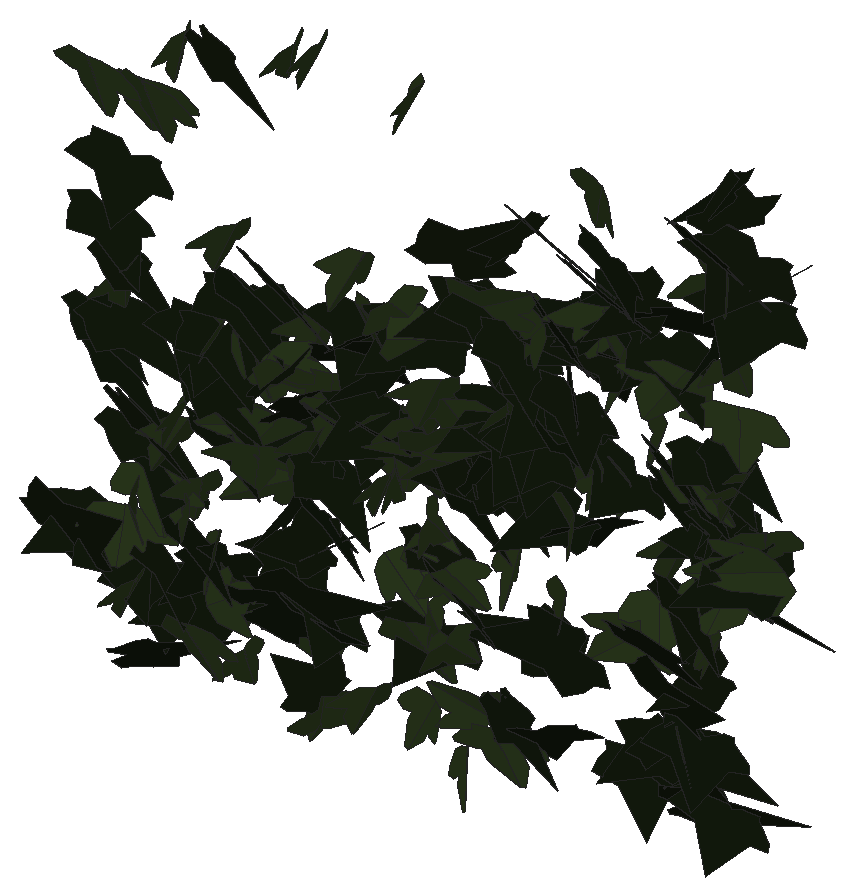
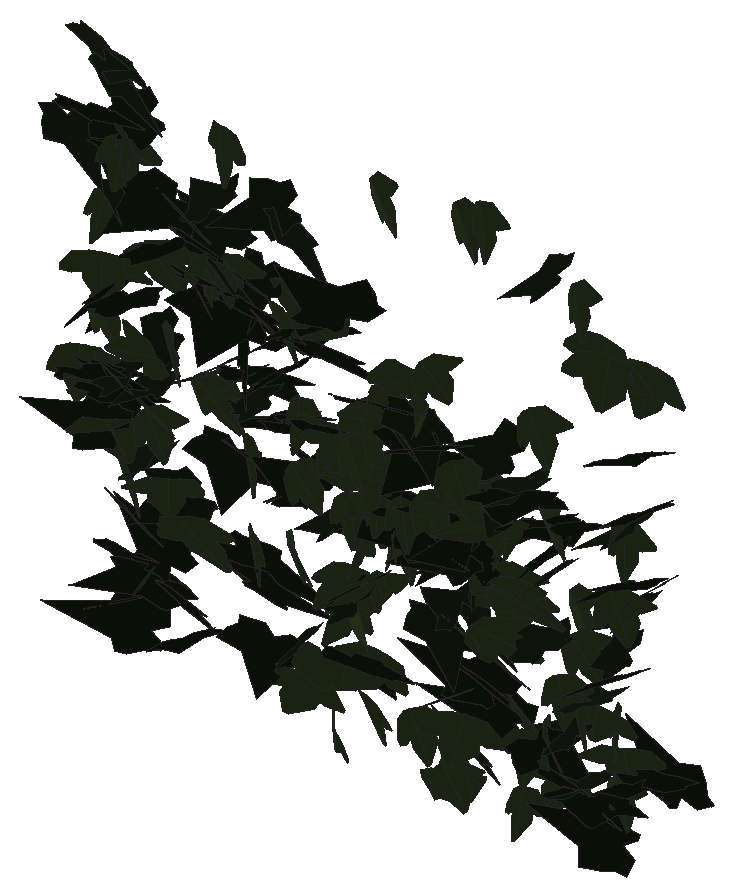
# SketchUp Ruby script. Lengths in millimetres.
U = 1.mm
M = Sketchup.active_model
def pt(a) = Geom::Point3d.new(a.map { |v| v * U })
def face(e, loops, mat)
  f = e.add_face(loops[0].map { |a| pt(a) })
  loops[1..].each { |l| e.add_face(l.map { |a| pt(a) }).erase! }
  f.material = f.back_material = mat if mat
  f
end
# faces: each face lists its corners as indices into pts; further lists are holes
def faces(e, pts, list, mat = nil) = list.each { |f| face(e, (f[0].is_a?(Array) ? f : [f]).map { |l| l.map { |i| pts[i] } }, mat) }
# xy, xz, yz: faces in a plane at the given z, y or x. An outline is a flat list of corners, or four numbers for a rectangle; further outlines are holes
def ring(l) = l.size == 4 ? [[l[0], l[1]], [l[2], l[1]], [l[2], l[3]], [l[0], l[3]]] : l.each_slice(2).to_a
def flat(e, list, mat, &to3) = list.each { |f| face(e, (f[0].is_a?(Array) ? f : [f]).map { |l| ring(l).map { |u, v| to3.(u, v) } }, mat) }
def xy(e, z, list, mat = nil) = flat(e, list, mat) { |x, y| [x, y, z] }
def xz(e, y, list, mat = nil) = flat(e, list, mat) { |x, z| [x, y, z] }
def yz(e, x, list, mat = nil) = flat(e, list, mat) { |y, z| [x, y, z] }
def lines(e, pts, list) = list.each { |a, b| e.add_line(pt(pts[a]), pt(pts[b])) }
# prism: a flat outline (further loops are holes) pulled along v
def prism(e, loops, v, mat = nil)
  f = face(e, loops, mat); d = Geom::Vector3d.new(v.map { |x| x * U })
  f.pushpull(f.normal.samedirection?(d) ? d.length : -d.length)
end
def box(e, o, s, mat = nil) = prism(e, [[o, [o[0] + s[0], o[1], o[2]], [o[0] + s[0], o[1] + s[1], o[2]], [o[0], o[1] + s[1], o[2]]]], [0, 0, s[2]], mat)
def at(x, y, z, deg = 0) = Geom::Transformation.translation(pt([x, y, z])) * Geom::Transformation.rotation(ORIGIN, Z_AXIS, deg.degrees)
def axes(o, x, y, z) = Geom::Transformation.new([*x, 0, *y, 0, *z, 0, *pt(o).to_a, 1])
def part(name) = M.definitions.add(name)
# library, detail: a bought-in or finely detailed component or shape, given as its bounding box
def library(name, o, s) = part(name).tap { |d| box(d.entities, o, s) }
def detail(e, o, s) = box(e.add_group.entities, o, s)
def put(e, d, t, mat = nil) = e.add_instance(d, t).tap { |i| i.material = mat if mat }
def group(e, t, mat = nil) = e.add_group.tap { |g| g.transformation = t; g.material = mat if mat }.entities
root = M.entities
M.materials.add("efeu1").color = [18, 25, 13]
M.materials.add("efeu2").color = [43, 57, 29]
c1 = part("ivyleaf_9")
p = [[39.1,54.8,31.7],[34.5,51.8,30.2],[-5.3,25.2,17.3],[-17.9,28.3,20.9],[-21.6,21.7,17],[-20.2,4.3,5.3],
  [-22.9,-0.3,2.5],[-17.1,-4,-0.6],[-2,-2.1,-1.2],[-0.7,-15.4,-10.1],[16.6,-22.3,-16.7],[21.1,-15.1,-12.5],
  [32.7,-10.7,-11],[46.1,-1.8,-6.6],[30.8,11.2,3.8]]
faces(c1.entities,p,[[0,1,2,3,4,5,6,7,8,9,10,11,12,13,14]],"efeu1")
c2 = part("ivyleaf_10")
p = [[0,12.8,-0.8],[-1.5,51.3,-10.9],[-4.9,51,-11.6],[-13.6,26.5,-7.3],[-13.2,15.9,-4.6],[-21.1,19.3,-7.2],
  [-29.5,16.3,-8.3],[-29.2,8.3,-6.2],[-19.7,-9.8,0.5],[-7.6,-13,4],[1,-12.2,5.8],[-0.4,51.1,-11.1],
  [-1.5,51.1,-10.9],[1,-12.4,5.9],[16.9,-12.4,3.5],[35.1,9.1,-5.1],[35,12.9,-6.1],[20.5,16.4,-4.9],
  [15.8,15,-3.8],[15.3,27.6,-7.1],[12.8,31.3,-7.8]]
faces(c2.entities,p,[[0,1,2,3,4,5,6,7,8,9,10],[11,12,0,13,14,15,16,17,18,19,20]],"efeu2")
put(root,c1,axes([4004.6,807.1,2723.3],[-1.72349,-0.38315,0.30559],[-0.51909,-0.13943,-0.98307],[0.77495,-0.94552,0.02113]))
put(root,c1,axes([3962.3,785.5,2704.8],[-0.47252,0.12478,1.19338],[1.21455,-1.01828,0.23923],[1.93387,0.67001,0.14134]))
put(root,c2,axes([4006,787.8,3291.4],[-2.04812,0.34445,-0.02824],[0.02425,-0.05275,-1.12898],[-0.65731,-1.07522,0.04634]))
put(root,c1,axes([3997.3,798.5,2991.7],[0.61956,-0.96621,-0.38496],[-0.14432,0.38025,-1.01852],[1.97419,0.33102,0.04636]))
put(root,c1,axes([4005.8,810.3,3106.3],[-0.00206,-1.09219,-0.16823],[0.07466,0.16809,-1.0915],[2.10184,-0.00704,0.03861]))
put(root,c2,axes([4038.1,819,2966.8],[-0.79231,-1.00282,0.18365],[0.00996,-0.20047,-1.08281],[1.94029,-0.40847,0.08055]))
put(root,c1,axes([4033.7,814.1,3176.8],[-0.91795,-0.98023,0.18834],[0.03143,-0.21698,-1.08702],[1.89944,-0.47013,0.109]))
put(root,c1,axes([4023.4,804,2703.1],[-0.20194,-1.01434,-0.32948],[0.12304,0.32438,-1.01946],[2.02605,-0.1208,0.02907]))
put(root,c2,axes([4035.6,801.1,2740.4],[1.71839,0.57529,-0.10566],[-0.18811,-0.04148,-1.07045],[-1.0972,0.90811,0.01804]))
put(root,c2,axes([4044.9,789.4,3049.4],[-0.37987,-1.03459,-0.33106],[0.16608,0.32024,-1.0534],[2.06071,-0.21653,0.02387]))
put(root,c1,axes([4024.5,788.4,2950.3],[0.88277,-0.96056,-0.20735],[-0.12452,0.19859,-1.06635],[1.8661,0.46765,0.02693]))
put(root,c1,axes([4025,799.5,2992.3],[0.4837,-0.85668,-0.61589],[0.28995,0.65666,-0.85053],[1.98701,0.11272,0.27404]))
put(root,c2,axes([4061,781,2676.1],[-0.15705,-1.01305,-0.15562],[-0.00419,0.1563,-1.0163],[1.95065,-0.08123,-0.01471]))
put(root,c2,axes([4070.3,776.8,2773.9],[-0.55798,0.64958,0.78832],[-0.92662,0.63213,-0.70194],[-1.70902,-0.55481,0.12321]))
put(root,c1,axes([4032.1,793.5,3068.4],[1.03234,-0.93965,-0.3083],[-0.04797,0.33838,-1.07568],[1.88153,0.52419,0.14173]))
put(root,c1,axes([4037.2,812.7,2858.8],[0.73316,-0.85605,-0.58965],[0.11836,0.64669,-0.89823],[1.97478,0.27906,0.27275]))
put(root,c2,axes([4073.6,795.2,3286.1],[-2.13847,-0.12835,0.03775],[-0.07317,0.00396,-1.1309],[0.24389,-1.12425,-0.00829]))
put(root,c1,axes([4039,797.4,2886.7],[1.24053,-0.8578,0.06357],[0.06334,-0.05455,-1.07733],[1.63581,0.65263,-0.0065]))
put(root,c1,axes([4077.4,822,2674.8],[-1.29878,-0.72357,-0.43124],[0.56055,0.315,-0.99461],[1.50194,-0.74326,-0.0017]))
put(root,c2,axes([4070.1,810.4,2795.4],[2.02443,-0.08077,0.312],[0.59043,-0.03493,-1.06671],[0.16619,1.10796,-0.01088]))
put(root,c1,axes([4081.3,827.1,2809.1],[-0.63423,-0.84696,0.56115],[0.15184,-0.61055,-0.87415],[1.92765,-0.23057,0.25348]))
put(root,c2,axes([4093,775.9,3296.1],[-2.00794,0.43932,-0.03649],[0.05659,-0.02351,-1.1428],[-0.83708,-1.0554,0.01027]))
put(root,c1,axes([4064.9,779.3,2592.2],[0.91622,0.90677,-0.46551],[0.34977,0.42916,1.02603],[1.90809,-0.51408,0.03545]))
put(root,c2,axes([4106.6,807.1,2876],[-0.38013,-1.01756,0.40443],[-0.0116,-0.41007,-1.03475],[2.08395,-0.18789,0.06801]))
put(root,c1,axes([4084.4,828,2688],[-0.26892,-0.97988,0.5077],[0.22139,-0.52221,-0.97552],[2.08866,-0.07081,0.16877]))
put(root,c2,axes([4117.7,798.6,2786.9],[0.89494,-0.78912,-0.53773],[-0.22852,0.54577,-0.90592],[1.80297,0.46087,0.15209]))
put(root,c2,axes([4124.4,787.2,3367.2],[0.08101,-1.14133,-0.10536],[0.22551,0.10925,-1.13559],[2.16973,0.03126,0.12196]))
put(root,c2,axes([4130.4,779.9,2920.2],[0.32381,-1.08677,0.02998],[0.00989,-0.02953,-1.10001],[2.0691,0.17022,0.00056]))
put(root,c2,axes([4130.6,811.7,2811.8],[-0.61298,-0.98323,-0.10761],[0.13937,0.08916,-1.03381],[1.8773,-0.32767,0.04161]))
put(root,c1,axes([4162.6,808.7,2679.1],[-2.03173,0.36853,0.09714],[-0.17909,0.02508,-1.12933],[-0.70289,-1.07165,0.00698]))
put(root,c1,axes([4109.2,813.4,2750.4],[0.60615,-1.00713,0.35708],[0.28831,-0.32628,-1.05539],[2.01314,0.34997,0.04363]))
put(root,c1,axes([4159.8,821.7,2725.4],[0.03041,0.38777,-0.98513],[0.05152,-0.98507,-0.38731],[-2.01427,-0.01934,-0.02478]))
put(root,c2,axes([4140,825.9,2736.1],[0.822,-0.72874,0.63942],[0.68113,-0.53071,-0.84659],[1.71481,0.56012,0.02976]))
put(root,c2,axes([4154.2,772,2652.5],[-1.80375,0.35185,-0.20836],[0.38987,-0.04667,-1.01059],[-0.67355,-0.96926,-0.02698]))
put(root,c1,axes([4163.6,791.5,3019.6],[-1.04671,-0.97554,0.10136],[-0.08043,-0.09253,-1.11985],[1.86491,-0.55153,0.00859]))
put(root,c2,axes([4173.8,786.2,3028.6],[0.66739,-1.03691,0.10548],[0.03954,-0.10431,-1.09452],[1.98324,0.35102,-0.01367]))
put(root,c1,axes([4146.9,827,2868.1],[0.20036,-0.89986,0.58289],[0.55983,-0.53898,-0.8852],[1.96223,0.24566,0.19303]))
put(root,c1,axes([4156.9,799.4,2958.2],[0.59458,-1.02655,-0.16373],[-0.05627,0.16212,-1.07287],[1.97763,0.31325,0.0187]))
put(root,c2,axes([4186.3,809.2,2706],[-1.62772,0.5965,0.21832],[-0.3537,0.11515,-1.04266],[-1.156,-0.87514,0.01161]))
put(root,c2,axes([4196.7,782.2,3158.7],[-0.47503,-1.11575,0.00757],[-0.03301,-0.00388,-1.14322],[2.12329,-0.24968,-0.01608]))
put(root,c1,axes([4173.9,773.7,2978.9],[0.73145,-0.84348,-0.68833],[-0.52372,0.63099,-0.92687],[2.00473,0.4726,0.00901]))
put(root,c1,axes([4167.4,779.6,3380.1],[1.24893,-0.93043,-0.21111],[-0.17753,0.19243,-1.13805],[1.8071,0.66194,0.0341]))
put(root,c2,axes([4223.1,809.6,2917.5],[1.11307,-0.02398,-0.89333],[-1.67782,0.15942,-0.58143],[0.27863,1.05578,0.06751]))
put(root,c1,axes([4179.7,794.3,3025.8],[-0.34449,-1.03258,-0.32929],[0.19395,0.31616,-1.04741],[2.05357,-0.20308,0.04369]))
put(root,c2,axes([4195.2,807.4,2625.5],[-0.37053,-0.93343,-0.45534],[0.31577,0.42937,-0.95112],[1.95122,-0.24674,0.06745]))
put(root,c2,axes([4201,800.8,3014.6],[-0.16874,0.98331,0.40809],[-0.11719,0.40408,-0.98703],[-2.0228,-0.10544,0.02314]))
put(root,c2,axes([4183.5,784.2,2696.3],[1.13594,-0.66051,-0.63385],[0.96177,-0.39322,0.8856],[-1.45276,-0.77678,0.09067]))
put(root,c1,axes([4201.3,818.4,3066.6],[-0.83824,-0.94982,-0.47901],[0.36087,0.44005,-1.0469],[1.99214,-0.47937,-0.01192]))
put(root,c2,axes([4243.8,820.9,2852.3],[-0.67445,-0.45566,0.90524],[-0.912,-0.76968,-0.57501],[1.69957,-0.59383,0.05068]))
put(root,c1,axes([4196.4,812.5,3070.8],[0.21125,-1.03991,0.36563],[0.37035,-0.34322,-1.03525],[2.06497,0.16794,0.14827]))
put(root,c2,axes([4241.3,800.7,2929.6],[-1.41847,-0.64198,0.39704],[-0.43347,-0.3407,-0.97842],[1.36964,-0.77269,0.10154]))
put(root,c2,axes([4235.4,782.8,2897.6],[-1.58116,-0.65461,0.0091],[-0.0206,-0.00096,-1.05768],[1.24581,-0.83084,-0.00594]))
put(root,c2,axes([4224.1,804.7,2994.5],[-0.51811,1.02654,0.03381],[-0.04487,0.02873,-1.06191],[-1.95426,-0.27281,0.01542]))
put(root,c1,axes([4224.6,803,3109.4],[1.1001,-0.85402,0.42106],[0.42528,-0.35716,-1.03115],[1.76159,0.61956,-0.01401]))
put(root,c1,axes([4272.9,760.2,3009.2],[0.34895,0.71885,0.86475],[0.16911,0.86417,-0.73721],[-2.13349,0.18607,0.083]))
put(root,c1,axes([4280,804.1,2773.1],[-1.85259,0.08254,-0.36864],[0.66451,-0.19245,-0.96503],[-0.2745,-1.02293,0.15181]))
put(root,c2,axes([4249,796.6,2999.3],[-0.56324,-0.37462,-1.03871],[1.62579,0.60372,-0.46113],[1.3316,-0.89556,0.12365]))
put(root,c1,axes([4289.2,791.1,2856.6],[-1.10313,0.75082,-0.54968],[0.68561,-0.41604,-0.94814],[-1.63288,-0.68192,-0.02675]))
put(root,c1,axes([4321.7,799,2919.1],[-1.42097,0.60353,0.50151],[-0.94866,0.16988,-0.94652],[-1.15346,-0.88323,0.16064]))
put(root,c1,axes([4239.9,776.7,2707.5],[0.93031,-0.16923,0.92241],[1.6381,-0.33207,-0.51704],[0.7087,0.9897,-0.01575]))
put(root,c2,axes([4288.6,771.4,3421.1],[-0.11345,-1.05176,-0.41149],[0.04644,0.41077,-1.05345],[2.14895,-0.0644,0.00104]))
put(root,c1,axes([4261.5,794.8,2954.1],[1.05481,0.4218,0.90625],[1.28884,0.60377,-0.69516],[-1.39935,0.87403,0.04286]))
put(root,c2,axes([4294.9,816.5,3064.8],[-0.79444,-1.01685,0.1269],[0.05064,-0.14773,-1.09627],[1.94963,-0.41051,0.08019]))
put(root,c1,axes([4324.3,782.2,2815.5],[-1.50442,0.63904,0.28154],[-0.47543,0.13833,-1.01535],[-1.24108,-0.82763,0.04768]))
put(root,c2,axes([4275.8,769.1,3032],[-0.70048,-0.47773,-0.92398],[1.19831,0.67784,-0.60127],[1.57578,-0.72783,0.04651]))
put(root,c2,axes([4296.6,807.4,2695],[-1.76895,-0.55922,-0.16061],[0.27815,0.06859,-1.0846],[1.07183,-0.94074,0.01639]))
put(root,c2,axes([4301.4,791.9,2935.8],[-0.19547,-1.03555,0.19862],[-0.00042,-0.19953,-1.04046],[2.00679,-0.10091,0.01913]))
put(root,c2,axes([4309.5,789.7,3420.6],[0.16584,-1.14167,-0.01643],[-0.00296,0.01636,-1.14499],[2.17306,0.08715,-0.00031]))
put(root,c1,axes([4338.8,759.4,2648.6],[-0.37466,0.78352,0.69383],[-0.62673,0.62377,-0.79783],[-1.89066,-0.36204,0.12698]))
put(root,c2,axes([4321.1,803.8,3007.9],[-1.6898,-0.6538,0.00865],[0.00491,-0.0181,-1.1025],[1.24441,-0.88773,0.0161]))
put(root,c2,axes([4320.1,803.9,2615],[-0.55887,-0.9536,0.29057],[-0.00519,-0.30214,-0.99434],[1.89726,-0.28172,0.08287]))
put(root,c2,axes([4317.2,794.3,2590.9],[-0.7593,-1.01832,-0.25647],[-0.18173,-0.23804,1.09368],[-1.99031,0.41022,-0.00202]))
put(root,c1,axes([4284.7,814.5,2950.5],[1.81736,-0.45932,0.18687],[0.36764,-0.02888,-1.0581],[0.86921,0.97258,0.05683]))
put(root,c1,axes([4282.1,772.8,2737.1],[0.28625,-0.11983,1.045],[1.91914,-0.28394,-0.17769],[0.5696,1.01687,0.07353]))
put(root,c1,axes([4320.9,806,2725.9],[-0.65001,-0.89249,0.46777],[-0.07837,-0.48113,-0.94806],[1.91615,-0.32244,0.1199]))
put(root,c1,axes([4342.7,793.5,2822.4],[0.06682,1.09872,0.11527],[-0.00645,0.11544,-1.09926],[-2.10255,0.03457,0.00704]))
put(root,c2,axes([4351.2,800.2,2973.9],[-1.76305,-0.28371,0.44612],[-0.76322,-0.20944,-0.96591],[0.65571,-1.00663,0.07523]))
put(root,c1,axes([4313.5,794.8,2846.2],[0.43636,-0.85207,0.62346],[0.4154,-0.58595,-0.88108],[1.96599,0.31293,0.04779]))
put(root,c1,axes([4329.1,783.5,2912.8],[0.20382,-1.02724,-0.36339],[-0.01766,0.36426,-1.03246],[2.0737,0.10407,0.02693]))
put(root,c1,axes([4358.6,822.6,3079.8],[-1.13295,-0.88266,0.24229],[0.05544,-0.30715,-1.04736],[1.74114,-0.56456,0.191]))
put(root,c2,axes([4363.8,789,3175.7],[-0.36732,-0.96134,0.57087],[0.1721,-0.59084,-0.96439],[2.12093,-0.11855,0.17712]))
put(root,c1,axes([4352,788.8,3064.8],[1.7097,0.62592,0.15329],[0.25691,0.07438,-1.09477],[-1.19924,0.90827,-0.01599]))
put(root,c1,axes([4388.2,781.1,3099.9],[0.10001,1.09647,0.03541],[0.00491,0.03532,-1.09773],[-2.08789,0.0526,-0.00089]))
put(root,c2,axes([4376.4,792.1,3113.8],[-0.9993,0.94034,0.09055],[-0.05385,0.0879,-1.07685],[-1.79712,-0.52551,-0.01808]))
put(root,c2,axes([4384.8,813.5,2979.4],[-0.53827,-1.02643,-0.11188],[0.10284,0.10113,-1.06438],[1.96237,-0.28685,0.02509]))
put(root,c1,axes([4381,816.1,2983.1],[-1.09656,-0.91367,0.00551],[0.00145,-0.007,-1.08016],[1.73893,-0.57615,0.00438]))
put(root,c1,axes([4404.4,804.7,2984.8],[-1.83572,-0.43895,0.26583],[-0.439,-0.13473,-1.0594],[0.87245,-0.99139,0.02627]))
put(root,c2,axes([4390.8,781.3,2657.1],[-0.52573,-1.05716,0.09692],[-0.02393,-0.09688,-1.09258],[2.02028,-0.27625,0.01228]))
put(root,c2,axes([4402.9,792,2921.4],[-0.03009,-1.0904,-0.1279],[0.025,0.12772,-1.09045],[2.08932,-0.01723,0.0112]))
put(root,c1,axes([4364.3,805.2,2952.8],[1.84249,-0.29411,0.40294],[0.72125,-0.13848,-1.01158],[0.61744,1.03943,-0.02076]))
put(root,c1,axes([4423.2,779.9,3074.7],[-1.48501,0.65891,-0.36536],[0.43797,-0.29242,-1.01883],[-1.3654,-0.81043,0.07056]))
put(root,c2,axes([4418.3,787.7,2932.1],[0.36696,-0.88227,-0.62108],[0.23073,0.64464,-0.8781],[2.04046,0.08578,0.21099]))
put(root,c2,axes([4422.4,811.8,2987.9],[-0.6003,-1.02853,-0.2291],[0.35173,0.18144,-1.069],[1.97438,-0.34504,0.12078]))
put(root,c2,axes([4435.2,795.9,2962.8],[-1.62528,-0.65551,0.03164],[-0.04665,-0.02003,-1.07656],[1.24816,-0.85433,0.00096]))
put(root,c2,axes([4424.2,781.3,3147.3],[-0.62579,-0.84895,-0.72925],[0.72933,0.62872,-0.90471],[2.00124,-0.4946,0.10167]))
put(root,c2,axes([4440.3,794,3411.3],[0.43885,-1.1117,0.0903],[0.01547,-0.09053,-1.13531],[2.1227,0.2305,-0.0104]))
put(root,c1,axes([4455,811.4,3109.6],[-1.95016,-0.36465,0.15589],[-0.07115,-0.34117,-1.04376],[0.75139,-0.97871,0.30576]))
put(root,c2,axes([4435.6,804.5,2737.5],[-1.86857,0.10934,-0.37482],[0.70839,-0.04422,-0.98787],[-0.22442,-1.04999,0.00257]))
put(root,c1,axes([4456,824.5,2744.2],[-1.94395,-0.32738,-0.21895],[0.40906,0.04662,-1.07239],[0.62812,-1.04357,0.02078]))
put(root,c2,axes([4437.4,766.9,2836.3],[0.35612,1.04272,0.37326],[0.14207,0.36581,-1.05934],[-2.10302,0.20128,-0.00836]))
put(root,c2,axes([4430.3,781.5,3110.8],[-0.13497,-0.29719,-1.1275],[1.20074,0.94017,-0.2875],[1.86625,-0.6264,0.10343]))
put(root,c2,axes([4450.6,811.8,2845.7],[0.69226,0.91566,-0.48714],[-0.44181,-0.43126,-0.98395],[-1.92388,0.42851,0.05067]))
put(root,c2,axes([4463.8,786.6,2661.8],[1.34814,-0.80223,-0.06363],[-0.06837,0.05316,-1.07018],[1.53008,0.70922,0.00824]))
put(root,c2,axes([4468.6,811.9,2956],[-0.71056,-0.99679,-0.16906],[0.09711,0.16141,-1.06438],[1.92172,-0.37672,-0.00872]))
put(root,c2,axes([4469.7,811.2,3033.6],[-0.23663,-1.07799,0.00508],[-0.00564,-0.00478,-1.08514],[2.05165,-0.12435,-0.0024]))
put(root,c1,axes([4448.6,818.9,2849.6],[0.35554,-1.02407,-0.26807],[-0.06305,0.26642,-1.04087],[2.0137,0.18916,0.01474]))
put(root,c2,axes([4453.8,812.7,2768.2],[-0.24817,-0.28105,-1.01183],[0.46518,-0.99972,0.24619],[-1.94373,-0.20337,0.18811]))
put(root,c2,axes([4480.1,780.5,3067],[-0.77467,-1.02802,0.13133],[-0.04636,-0.13157,-1.10537],[1.97188,-0.40696,0.02561]))
put(root,c2,axes([4469.6,783.5,2896.5],[0.24606,-0.7996,-0.73511],[0.39298,0.74489,-0.77393],[2.02949,-0.04729,0.23899]))
put(root,c1,axes([4461.5,815.2,2819.2],[0.83529,-0.90996,0.32836],[0.25023,-0.30112,-1.01021],[1.82406,0.45801,-0.01178]))
put(root,c2,axes([4475.1,787.5,2985.4],[-1.1698,-0.86358,0.47137],[0.7646,0.28705,1.04975],[-1.70925,0.71944,0.14698]))
put(root,c2,axes([4488.9,797.4,3037.2],[-1.82472,-0.35925,-0.34635],[0.5923,0.15595,-1.02327],[0.7424,-1.0074,-0.03489]))
put(root,c1,axes([4534.1,812.3,3161.2],[-2.03918,0.01709,0.23497],[-0.4482,-0.10751,-1.06606],[0.01222,-1.09163,0.10867]))
put(root,c2,axes([4495.5,791,2836.1],[-0.93617,-0.76298,-0.56099],[0.8343,0.37691,-0.89699],[1.59766,-0.6439,0.13969]))
put(root,c1,axes([4482.5,813.5,2934.5],[0.96981,-0.93877,-0.00238],[-0.01638,-0.00196,-1.06812],[1.7866,0.50957,-0.0085]))
put(root,c2,axes([4539.4,791.6,2680.4],[-1.0312,-0.40201,-0.81581],[-1.28021,-0.46199,0.6744],[-1.16497,0.86353,-0.01899]))
put(root,c1,axes([4491.5,800.6,3217.6],[-0.49372,-0.18547,1.1415],[2.12377,0.26703,0.29698],[-0.57791,1.13975,0.11618]))
put(root,c2,axes([4515.6,761.1,2770.9],[-0.58109,-0.73883,-0.79186],[0.50982,0.74564,-0.79899],[1.99714,-0.40532,-0.02644]))
put(root,c2,axes([4504.3,798.8,2609],[0.88081,-0.69474,0.60133],[0.82932,-0.42682,-0.82849],[1.53958,0.62738,0.10226]))
put(root,c1,axes([4564.3,786.5,2978.7],[-1.65701,0.54795,0.31794],[-0.53313,0.15171,-1.02853],[-1.08143,-0.91438,0.01988]))
put(root,c2,axes([4545.3,822.8,2976.5],[-0.25376,-1.0273,0.35616],[-0.01564,-0.35787,-1.03529],[2.06926,-0.12868,0.03585]))
put(root,c1,axes([4565.4,819.2,3040.6],[-1.84135,-0.39914,0.31593],[-0.45591,-0.24168,-1.03894],[0.85482,-0.98867,0.12642]))
put(root,c1,axes([4548,804.1,3177.6],[-0.82979,-1.00908,-0.14598],[0.06466,0.1443,-1.09894],[1.9394,-0.43655,-0.02582]))
put(root,c2,axes([4559.4,802.4,3058.5],[-0.23611,-0.947,-0.52897],[0.20561,0.51899,-0.95446],[2.05418,-0.16079,0.03473]))
put(root,c1,axes([4538.6,821.3,2963.4],[0.40935,-1.04062,-0.19521],[0.07583,0.20701,-1.05963],[2.01362,0.20375,0.07959]))
put(root,c2,axes([4552.6,823.3,2863],[1.11094,-0.84431,0.41919],[0.49358,-0.33018,-1.02618],[1.72482,0.6383,0.02366]))
put(root,c2,axes([4540.6,791.8,3180],[-1.55017,-0.38997,0.63527],[1.1877,0.1579,0.89705],[-0.77591,1.02081,0.10393]))
put(root,c1,axes([4544.9,800.2,2947],[-0.25923,-0.13847,1.15186],[1.82661,0.63812,0.1902],[-1.24048,0.96858,0.03936]))
put(root,c2,axes([4559.5,791.1,2657],[-1.85196,-0.14751,-0.26125],[0.53684,-0.14773,-0.96721],[0.19453,-0.99665,0.18204]))
put(root,c1,axes([4605.2,771.6,3296.6],[-0.80251,1.02341,0.04885],[-0.03742,0.04474,-1.10688],[-1.94962,-0.42212,0.00114]))
put(root,c1,axes([4570.3,815.3,3119.8],[0.58011,-0.93347,-0.48956],[-0.17244,0.48453,-0.98029],[1.99866,0.31275,0.05752]))
put(root,c1,axes([4633.6,803.6,2782.7],[-1.03639,0.37526,0.80588],[-1.33305,0.40084,-0.65995],[-1.04185,-0.88618,0.04275]))
put(root,c1,axes([4574.2,781.3,2705.4],[0.94663,-0.96584,-0.32269],[-0.32624,0.2746,-1.08609],[1.91042,0.52548,-0.02557]))
put(root,c2,axes([4605.9,792.2,3177.4],[1.16619,-0.85068,-0.41943],[-0.38324,0.37129,-1.04721],[1.76397,0.64307,0.04978]))
put(root,c1,axes([4584,794.6,3153.1],[-0.20204,-1.11959,-0.02287],[-0.03869,0.02489,-1.12438],[2.13089,-0.1057,-0.02258]))
put(root,c1,axes([4604.5,799.1,3029.6],[-1.38392,-0.78363,0.18193],[0.01391,-0.25166,-1.05477],[1.531,-0.70606,0.17403]))
put(root,c1,axes([4609.8,805.3,3029.6],[-0.82018,-1.00679,0.13133],[-0.07448,-0.12609,-1.09506],[1.93092,-0.43251,0.01354]))
put(root,c1,axes([4637,808.3,3086.4],[-1.82016,-0.53642,0.08761],[-0.14859,-0.0399,-1.09653],[1.02371,-0.95954,-0.00339]))
put(root,c1,axes([4623.7,779.5,2693],[1.07986,0.86405,-0.07424],[-0.05643,-0.06934,-1.03361],[-1.64956,0.56801,-0.01324]))
put(root,c1,axes([4669.8,783.2,2807.9],[-0.3726,-0.08532,-1.1826],[-2.03781,-0.5021,0.21348],[-0.96924,1.08847,0.00578]))
put(root,c1,axes([4652.1,801.6,2960.3],[-2.01531,0.20526,-0.12121],[0.16102,-0.19235,-1.06487],[-0.42414,-1.04832,0.17166]))
put(root,c2,axes([4629.9,808.3,2846.4],[0.91887,-0.92419,-0.24784],[0.09191,0.30078,-1.02755],[1.81875,0.45172,0.17714]))
put(root,c1,axes([4664.7,812.5,3183.4],[-2.10946,0.10615,0.0495],[-0.09441,0.0012,-1.11344],[-0.20192,-1.10948,0.00353]))
put(root,c1,axes([4612.5,808.6,3059.4],[1.19147,-0.92533,-0.04327],[0.07303,0.07809,-1.11466],[1.7615,0.62265,0.07548]))
put(root,c1,axes([4611.1,773.4,3318.9],[1.89651,-0.57605,-0.01614],[0.06985,0.0956,-1.14655],[1.09453,0.99202,0.10113]))
put(root,c1,axes([4648.3,767.9,3214.1],[1.47871,-0.16809,-0.88948],[-1.58997,0.31824,-0.78988],[0.66342,1.13735,0.08955]))
put(root,c1,axes([4663.4,788.4,3119.7],[0.5243,-0.14363,-1.1693],[-1.94467,0.56856,-0.31057],[1.11598,1.05825,0.00816]))
put(root,c2,axes([4656,787.4,2964.1],[0.96419,-0.84234,-0.59089],[-0.15119,0.62465,-0.95857],[1.95241,0.46436,0.21758]))
put(root,c1,axes([4644.2,819.9,3077.7],[0.28734,-1.08925,-0.05382],[0.00015,0.05434,-1.09964],[2.0756,0.15079,0.00753]))
put(root,c1,axes([4690.7,800,3214.1],[-1.43987,0.80612,-0.11843],[0.17396,-0.07662,-1.10544],[-1.54088,-0.76192,-0.01413]))
put(root,c1,axes([4670.3,795.1,2954.1],[0.82892,1.00029,0.08354],[0.07805,0.07325,-1.09097],[-1.90879,0.43739,-0.00833]))
put(root,c1,axes([4654.1,805.4,3102.4],[-0.19871,-1.09457,0.22286],[0.0232,-0.22493,-1.09904],[2.12579,-0.09986,0.03282]))
put(root,c1,axes([4676.1,802.9,3163.3],[1.84598,0.42082,-0.32376],[-0.58966,-0.09898,-1.05683],[-0.82062,1.01774,0.03109]))
put(root,c2,axes([4698,779.9,3040.4],[0.77721,-0.76687,-0.71557],[-0.55188,0.65542,-0.86789],[1.91841,0.49923,0.04023]))
put(root,c2,axes([4693.2,800.1,3219.6],[-1.45058,-0.8262,0.11751],[0.22508,-0.26448,-1.09243],[1.57221,-0.72442,0.26481]))
put(root,c2,axes([4716.2,795.1,3030.8],[0.86446,-0.26332,-1.00179],[-1.19991,0.79762,-0.49551],[1.56412,0.75742,0.17354]))
put(root,c1,axes([4740.1,799.4,3182.3],[-1.58914,0.51325,0.55525],[-1.11433,0.08455,-0.95862],[-0.91059,-0.99918,0.2041]))
put(root,c2,axes([4688.2,805.7,3212.9],[-1.48264,0.62595,-0.49887],[0.62036,-0.38771,-0.99549],[-1.39134,-0.8399,0.08774]))
put(root,c2,axes([4706.2,775.2,3387.1],[1.45599,-0.75814,-0.39913],[0.04111,0.55198,-1.00707],[1.63012,0.66324,0.38189]))
put(root,c1,axes([4741.7,805,3242.7],[-1.92013,0.46511,0.16794],[-0.35417,-0.00357,-1.10804],[-0.87195,-1.02277,0.08024]))
put(root,c2,axes([4729.9,816.4,2834.1],[1.73961,0.05653,-0.56273],[-1.07615,0.11302,-0.9071],[0.02181,1.06741,0.12585]))
put(root,c1,axes([4686.6,798.1,3252.3],[0.11119,-0.6431,0.92015],[1.01033,-0.79604,-0.59007],[1.88258,0.4652,0.26233]))
put(root,c2,axes([4722,798,3201.6],[1.1337,-0.95404,-0.14236],[0.06087,0.18676,-1.11776],[1.83483,0.58329,0.12504]))
put(root,c1,axes([4708.1,797.3,3297.1],[0.08701,-0.88476,0.68803],[0.29172,-0.6772,-0.88102],[2.11307,0.12992,0.0933]))
put(root,c2,axes([4731.4,795.3,3172.3],[0.91046,-1.02157,0.13207],[0.08275,-0.12546,-1.12795],[1.95868,0.48016,-0.01374]))
put(root,c1,axes([4737.1,801.1,3039.1],[-1.06813,-0.72343,0.59695],[-0.2254,-0.63543,-0.88141],[1.77077,-0.51726,0.24788]))
put(root,c1,axes([4735.1,819.1,2672.4],[-0.43923,-1.0318,0.01328],[-0.01957,-0.01131,-1.05727],[1.9638,-0.23089,-0.00757]))
put(root,c1,axes([4771.2,791.6,3272.5],[-1.86696,0.50498,-0.31046],[0.47071,-0.19688,-1.1017],[-1.02529,-1.0099,0.05954]))
put(root,c2,axes([4761.1,815.2,3095.9],[0.78692,-1.00666,-0.21323],[0.00333,0.23049,-1.08474],[1.95838,0.40411,0.08753]))
put(root,c1,axes([4782.2,800.5,2721.9],[-1.8771,0.24341,-0.15942],[0.27245,-0.08457,-1.01478],[-0.48211,-0.9955,0.04723]))
put(root,c2,axes([4762.9,814.5,2882.2],[1.5022,0.73186,-0.06208],[-0.08687,-0.04207,-1.07639],[-1.39518,0.79062,0.00018]))
put(root,c1,axes([4749.8,781,2856.3],[1.99335,-0.14747,-0.01146],[-0.01887,0.01174,-1.05765],[0.28087,1.04736,0.01024]))
put(root,c2,axes([4790,815.8,2966.7],[-0.50319,-1.06404,0.17978],[0.0372,-0.18979,-1.09454],[2.05345,-0.2573,0.06388]))
put(root,c2,axes([4809.4,787.6,3189.1],[-1.50626,-0.64485,0.49543],[-0.40812,-0.50137,-0.99514],[1.49288,-0.78769,0.22782]))
put(root,c1,axes([4773.2,804.4,3038.7],[1.55032,-0.60055,-0.42224],[-0.47421,0.36711,-1.00282],[1.31427,0.84087,0.13625]))
put(root,c1,axes([4765.4,812.3,2769.2],[0.07739,-0.17586,1.17807],[1.06128,-1.03879,-0.17432],[2.00318,0.55714,0.04684]))
put(root,c1,axes([4784.8,804.3,3216.8],[-0.1586,-1.04976,-0.39497],[0.03185,0.39486,-1.05297],[2.1344,-0.0839,-0.01364]))
put(root,c1,axes([4783.7,787.2,3083],[1.71282,-0.56662,-0.40796],[-0.6357,0.23505,-1.0633],[1.1669,0.95975,0.01956]))
put(root,c1,axes([4791.2,773.9,3268.1],[1.77564,0.51149,0.33908],[0.47386,0.24845,-1.05986],[-1.06749,0.96109,0.09353]))
put(root,c1,axes([4802.4,815.4,2895.2],[-0.28744,-0.8563,0.65557],[-0.07031,-0.65747,-0.8673],[2.05128,-0.14253,0.06214]))
put(root,c2,axes([4806.9,799.5,2737.9],[-0.28153,0.92852,-0.42254],[0.1593,-0.41448,-0.9401],[-1.935,-0.16922,-0.01592]))
put(root,c1,axes([4798,806.2,2907.7],[0.54365,-0.99746,0.28965],[0.10105,-0.28599,-1.03722],[1.97421,0.28932,-0.02667]))
put(root,c1,axes([4844.2,810,2824.3],[-1.72335,0.50055,-0.20633],[0.30672,-0.13464,-1.0339],[-0.98369,-0.9189,0.0391]))
put(root,c1,axes([4791.5,798.1,2728.4],[0.30582,-0.27875,-1.05659],[1.04916,0.94278,-0.16489],[1.79568,-0.50336,0.27629]))
put(root,c2,axes([4794.5,815.4,3058.6],[0.93805,-0.14872,0.97755],[1.82786,-0.1878,-0.51281],[0.44763,1.07854,0.0455]))
put(root,c2,axes([4845.5,799.3,2872.8],[0.73015,-0.95223,-0.41096],[-0.26537,0.38684,-1.02651],[1.95593,0.40795,0.01414]))
put(root,c1,axes([4868.7,803.8,3010.5],[-1.52993,0.74194,0.08421],[-0.10815,0.06259,-1.09391],[-1.417,-0.80585,-0.00743]))
put(root,c1,axes([4836,798.1,2749.3],[-1.56128,-0.37482,-0.5348],[1.06163,0.04437,-0.88676],[0.64636,-0.97827,0.16468]))
put(root,c1,axes([4820.2,825.9,3028.9],[0.86716,-0.97493,0.12419],[0.07915,-0.11764,-1.07608],[1.86881,0.45737,-0.01205]))
put(root,c1,axes([4876.2,817.9,3014.6],[-2.05685,0.11662,0.08419],[-0.16346,-0.01134,-1.08681],[-0.21959,-1.08394,0.02043]))
put(root,c1,axes([4806.7,805.2,2655.2],[1.11591,-0.06134,0.94648],[1.80497,0.05196,-0.58415],[-0.02278,1.11216,0.07949]))
put(root,c2,axes([4855.1,789.1,3328.7],[-0.8616,-0.98841,-0.31281],[0.38927,0.24947,-1.08429],[1.93431,-0.49047,0.07887]))
put(root,c1,axes([4878.4,792,3440],[-1.13154,0.93192,-0.26403],[0.22578,-0.23741,-1.1051],[-1.82956,-0.60567,0.02692]))
put(root,c2,axes([4857.9,814.8,2933.8],[1.7268,0.52764,-0.28584],[-0.50853,-0.10875,-1.04886],[-1.02263,0.94504,0.0389]))
put(root,c1,axes([4863.3,815.6,2987.5],[-1.51917,-0.73064,-0.11885],[0.16667,0.08035,-1.08212],[1.39894,-0.80301,-0.00014]))
put(root,c1,axes([4829.3,777.7,3377.8],[1.92934,-0.51359,0.00329],[0.00282,-0.00435,-1.1364],[0.97747,1.01373,-0.00321]))
put(root,c1,axes([4848.7,789.7,3114.7],[0.08679,-0.92924,-0.64101],[-0.07755,0.63976,-0.93033],[2.1471,0.06067,-0.00769]))
put(root,c2,axes([4869.2,783.5,3337.2],[1.21232,-0.90546,-0.33003],[0.01332,0.39995,-1.08376],[1.83413,0.59559,0.22602]))
put(root,c1,axes([4866.3,805,2669.2],[-0.88252,-0.93315,0.25954],[-0.06147,-0.27269,-1.03814],[1.84236,-0.45609,0.08969]))
put(root,c1,axes([4878.2,788.4,3268.7],[-1.1611,0.54223,-0.7783],[0.99888,-0.57786,-0.81399],[-1.50377,-0.80251,0.06025]))
put(root,c1,axes([4889.5,825.9,3009.8],[-1.59477,-0.67647,0.18147],[-0.2884,-0.10116,-1.07679],[1.3014,-0.85138,-0.01625]))
put(root,c2,axes([4881.6,803.5,3158.2],[-1.93951,-0.47277,0.04115],[0.2827,-0.41036,-1.03599],[0.8578,-0.93371,0.43447]))
put(root,c2,axes([4890.1,793.5,3090.2],[-0.06299,-1.10707,0.13559],[0.01414,-0.13587,-1.10751],[2.12267,-0.03195,0.0114]))
put(root,c1,axes([4870.4,792.2,3122],[0.69911,-0.80974,-0.66246],[-0.43317,0.62344,-0.88825],[1.94344,0.43024,0.04033]))
put(root,c1,axes([4915.5,791.6,2978],[-2.02455,0.14027,0.07765],[-0.1578,-0.03535,-1.07199],[-0.26117,-1.06601,0.04576]))
put(root,c2,axes([4886.5,785.2,3240.8],[-0.48202,-1.02607,-0.4364],[0.49984,0.38003,-1.04595],[2.0624,-0.33192,0.1515]))
put(root,c1,axes([4906.5,752.8,3432.8],[0.72441,0.71752,0.80645],[-0.44785,0.88971,-0.68054],[-2.00499,0.06051,0.44338]))
put(root,c2,axes([4925.8,786.5,2992.6],[1.29931,-0.09238,-0.97578],[-1.8388,0.1367,-0.68891],[0.31393,1.18302,0.00341]))
put(root,c1,axes([4908.5,795.3,3368.6],[-2.0127,-0.3638,-0.23365],[0.47056,-0.00234,-1.11543],[0.67507,-1.08304,0.0809]))
put(root,c1,axes([4861.4,816.3,2930.2],[1.14966,-0.58681,0.68899],[1.21923,-0.30788,-0.82387],[1.21665,0.86303,0.17456]))
put(root,c2,axes([4910.2,809.9,3015.3],[-1.26749,-0.85574,-0.13899],[0.18526,0.10034,-1.08425],[1.63956,-0.67289,0.01507]))
put(root,c1,axes([4915.9,791.8,3315.6],[-1.77589,-0.62216,-0.23747],[0.53027,0.00657,-1.11198],[1.15117,-0.96283,0.14587]))
put(root,c1,axes([4936.2,798.6,3344.9],[-0.33431,1.11116,-0.12358],[0.02437,-0.12309,-1.12494],[-2.12766,-0.176,0.00653]))
